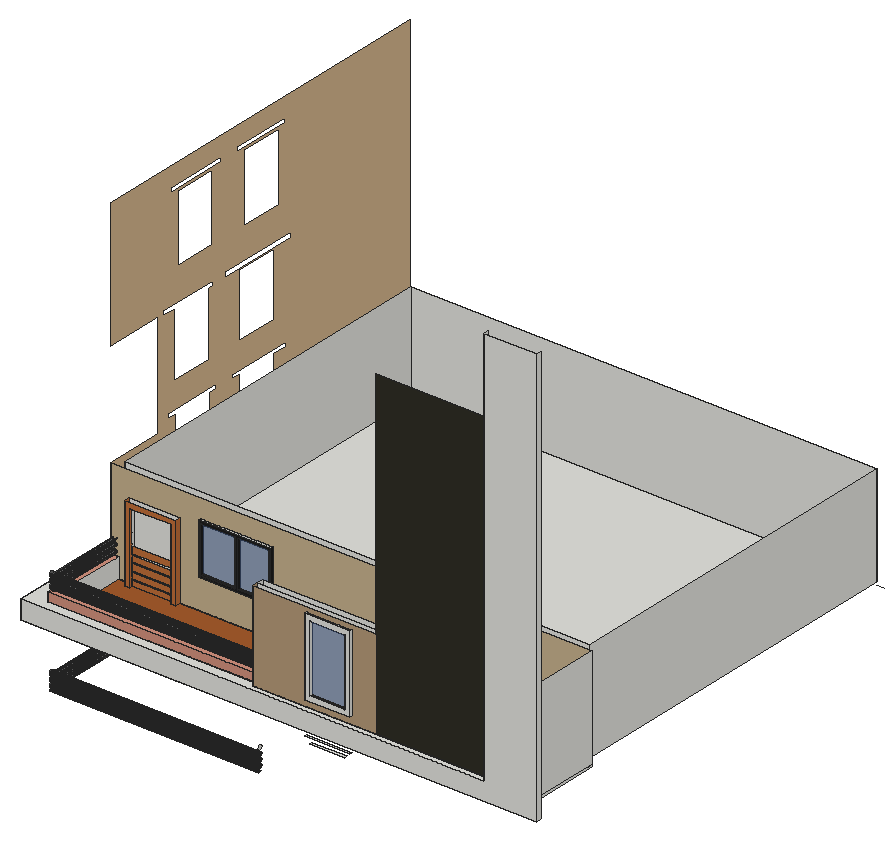
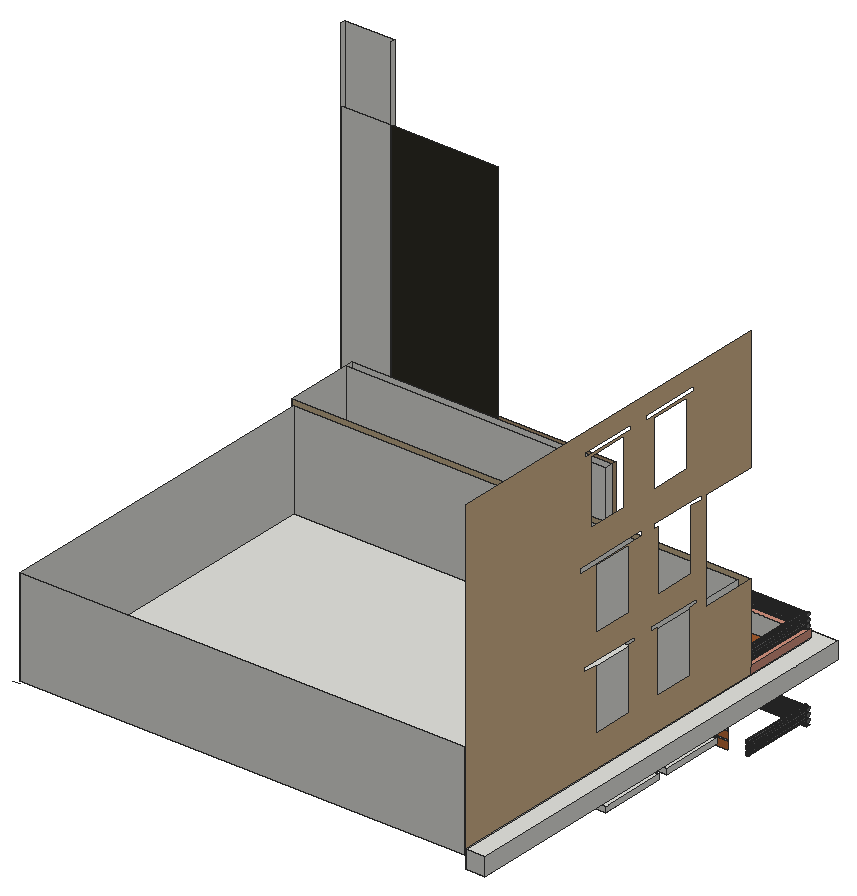
# SketchUp Ruby script. Lengths in inches.
U = 1.inch
M = Sketchup.active_model
def pt(a) = Geom::Point3d.new(a.map { |v| v * U })
def face(e, loops, mat)
  f = e.add_face(loops[0].map { |a| pt(a) })
  loops[1..].each { |l| e.add_face(l.map { |a| pt(a) }).erase! }
  f.material = f.back_material = mat if mat
  f
end
# faces: each face lists its corners as indices into pts; further lists are holes
def faces(e, pts, list, mat = nil) = list.each { |f| face(e, (f[0].is_a?(Array) ? f : [f]).map { |l| l.map { |i| pts[i] } }, mat) }
# xy, xz, yz: faces in a plane at the given z, y or x. An outline is a flat list of corners, or four numbers for a rectangle; further outlines are holes
def ring(l) = l.size == 4 ? [[l[0], l[1]], [l[2], l[1]], [l[2], l[3]], [l[0], l[3]]] : l.each_slice(2).to_a
def flat(e, list, mat, &to3) = list.each { |f| face(e, (f[0].is_a?(Array) ? f : [f]).map { |l| ring(l).map { |u, v| to3.(u, v) } }, mat) }
def xy(e, z, list, mat = nil) = flat(e, list, mat) { |x, y| [x, y, z] }
def xz(e, y, list, mat = nil) = flat(e, list, mat) { |x, z| [x, y, z] }
def yz(e, x, list, mat = nil) = flat(e, list, mat) { |y, z| [x, y, z] }
def lines(e, pts, list) = list.each { |a, b| e.add_line(pt(pts[a]), pt(pts[b])) }
# prism: a flat outline (further loops are holes) pulled along v
def prism(e, loops, v, mat = nil)
  f = face(e, loops, mat); d = Geom::Vector3d.new(v.map { |x| x * U })
  f.pushpull(f.normal.samedirection?(d) ? d.length : -d.length)
end
def box(e, o, s, mat = nil) = prism(e, [[o, [o[0] + s[0], o[1], o[2]], [o[0] + s[0], o[1] + s[1], o[2]], [o[0], o[1] + s[1], o[2]]]], [0, 0, s[2]], mat)
def at(x, y, z, deg = 0) = Geom::Transformation.translation(pt([x, y, z])) * Geom::Transformation.rotation(ORIGIN, Z_AXIS, deg.degrees)
def axes(o, x, y, z) = Geom::Transformation.new([*x, 0, *y, 0, *z, 0, *pt(o).to_a, 1])
def part(name) = M.definitions.add(name)
# library, detail: a bought-in or finely detailed component or shape, given as its bounding box
def library(name, o, s) = part(name).tap { |d| box(d.entities, o, s) }
def detail(e, o, s) = box(e.add_group.entities, o, s)
def put(e, d, t, mat = nil) = e.add_instance(d, t).tap { |i| i.material = mat if mat }
def group(e, t, mat = nil) = e.add_group.tap { |g| g.transformation = t; g.material = mat if mat }.entities
root = M.entities
M.materials.add("[0032_Moccasin]").color = [198, 177, 141]
M.materials.add("[0035_Tan]").color = [181, 154, 120]
M.materials.add("[0035_Tan]1").color = [210, 180, 140]
M.materials.add("[0134_DimGray]").color = [105, 105, 105]
M.materials.add("[Color B02]").color = [209, 145, 125]
M.materials.add("[Color M08]").color = [30, 30, 30]
M.materials.add("[Stone Coursed Rough]").color = [48, 46, 38]
M.materials.add("[Translucent Glass Blue]").color = [61, 91, 145]
M.materials["[Translucent Glass Blue]"].alpha = 0.5
M.materials.add("[Wood Square Tile 01]").color = [164, 91, 44]
M.materials.add("[Wood Veneer 01]").color = [191, 111, 58]
xy(root,456,[[66.43,116.9375,114.43,119.9375]])
xy(root,456,[[66.43,113.9375,114.43,116.9375]],"[Wood Veneer 01]")
xy(root,462,[[60.43,113.9375,120.43,119.9375]],"[Wood Veneer 01]")
xy(root,463.8125,[[144.33,116.9375,184.18,119.9375],[187.18,116.9375,224.02,119.9375]],"[Color M08]")
xy(root,464.8,[[31.875,212.29,34.875,264.41],[31.875,307.48,34.875,359.6]],"[Color M08]")
xy(root,466.8125,[[141.33,116.9375,227.02,119.9375]],"[Color M08]")
xy(root,470.15,[[352.1,17.9375,393.78,20.9375]])
xy(root,470.8,[[13.875,198.91,13.875,276.26,34.875,276.26,34.875,270.41,31.875,270.41,31.875,206.29,34.875,206.29,34.875,198.91],[13.875,289.66,13.875,372.1,34.875,372.1,34.875,365.6,31.875,365.6,31.875,301.48,34.875,301.48,34.875,289.66]])
xy(root,476.15,[[346.1,17.9375,399.78,20.9375]])
xy(root,477.3,[[13.875,198.91,34.875,276.26],[13.875,289.66,34.875,372.1]])
xy(root,483.875,[[11.5625,14.9375,11.5625,561.98,34.875,561.98,34.875,26.9375,282.125,26.9375,282.125,20.9375,623,20.9375,623,14.9375]])
xy(root,485.875,[[282.125,26.9375,604.125,35.9375]])
xy(root,489,[[34.875,26.9375,604.125,119.9375]])
xy(root,492,[[56.21,113.9375,62.21,119.9375],[110.21,113.9375,116.21,119.9375],[62.21,116.9375,110.21,119.9375],[43.875,128.9375,595.125,552.98]])
xy(root,492,[[43.875,35.9375,604.125,35.9375,604.125,119.9375,116.21,119.9375,116.21,113.9375,110.21,113.9375,110.21,116.9375,62.21,116.9375,62.21,113.9375,56.21,113.9375,56.21,119.9375,43.875,119.9375]],"[Wood Square Tile 01]")
xy(root,505.8125,[[11.5625,14.9375,561.08,14.9375,561.08,20.9375,282.125,20.9375,282.125,26.9375,34.875,26.9375,34.875,561.98,11.5625,561.98]])
xy(root,514.96,[[346.1,17.9375,399.78,20.9375]])
xy(root,516,[[282.125,26.9375,604.125,35.9375]])
xy(root,516,[[34.875,26.9375,282.125,26.9375,282.125,35.9375,43.875,35.9375,43.875,119.9375,34.875,119.9375]],"[Color B02]")
xy(root,520.96,[[352.1,17.9375,393.78,20.9375]])
xy(root,529.3125,[[141.33,116.9375,227.02,119.9375]])
xy(root,532.3125,[[144.33,116.9375,184.18,119.9375],[187.18,116.9375,224.02,119.9375]],"[Color M08]")
xz(root,14.9375,[[11.5625,483.875,623,483.875,623,980,561.08,980,561.08,505.8125,11.5625,505.8125]])
xz(root,17.9375,[[[346.1,514.96,399.78,606.77],[352.1,520.96,393.78,600.77]]])
xz(root,20.9375,[[282.125,483.875,623,492],[282.125,492,623,492,623,888,561.08,888,561.08,505.8125,282.125,505.8125],[[346.1,514.96,399.78,606.77],[352.1,520.96,393.78,600.77]]])
xz(root,20.9375,[[[282.125,505.8125,427.625,612],[346.1,514.96,399.78,606.77]]],"[0035_Tan]")
xz(root,20.9375,[[427.625,505.8125,561.08,888]],"[Stone Coursed Rough]")
xz(root,20.9375,[[352.1,520.96,393.78,600.77]],"[Translucent Glass Blue]")
xz(root,26.9375,[[34.875,483.875,282.125,489],[282.125,485.875,604.125,489],[34.875,489,282.125,505.8125],[282.125,489,604.125,492],[282.125,492,604.125,516],
  [282.125,516,604.125,612]])
xz(root,26.9375,[[34.875,505.8125,282.125,516]],"[Color B02]")
xz(root,29.17,[[37.22,519.63,41.83,519.63,41.9,520.15,41.82,520.76,41.78,520.86,37.27,520.86,37.23,520.76,37.15,520.15],[37.27,520.86,41.78,520.86,41.58,521.34,41.21,521.83,40.71,522.2,40.14,522.44,39.53,522.52,38.91,522.44,38.34,522.2,37.85,521.83,37.47,521.34]])
xz(root,29.17,[[39.53,517.77,40.14,517.85,40.71,518.09,41.21,518.47,41.58,518.96,41.82,519.53,41.83,519.63,37.22,519.63,37.23,519.53,37.47,518.96,37.85,518.47,38.34,518.09,38.91,517.85]],"[0134_DimGray]")
xz(root,35.9375,[[43.875,492,282.125,516],[282.125,492,604.125,516],[282.125,516,604.125,612]])
xz(root,113.9375,[[56.21,492,62.21,492,62.21,576,110.21,576,110.21,492,116.21,492,116.21,582,56.21,582]],"[Wood Veneer 01]")
xz(root,116.9375,[[66.43,419.66,114.43,421.37],[66.43,431.09,114.43,432.81],[66.43,442.53,114.43,444.25],[62.21,498.38,110.21,499.69],[62.21,507.45,110.21,508.75],
  [62.21,516.51,110.21,517.82],[62.21,525.57,110.21,526.88]])
xz(root,116.9375,[[[141.33,529.3125,227.02,590],[144.33,532.3125,184.18,587],[187.18,532.3125,224.02,587]]],"[Color M08]")
xz(root,116.9375,[[66.43,409.93,114.43,419.66],[66.43,421.37,114.43,431.09],[66.43,432.81,114.43,442.53],[66.43,444.25,114.43,456],[62.21,492,110.21,498.38],
  [62.21,499.69,110.21,507.45],[62.21,508.75,110.21,516.51],[62.21,517.82,110.21,525.57],[62.21,526.88,110.21,534.63]],"[Wood Veneer 01]")
xz(root,119.9375,[[56.21,486,116.21,489],[34.875,489,35.6,492],[35.6,489,56.21,492],[56.21,489,116.21,492],[116.21,489,604.125,492],
  [34.875,492,35.6,516],[35.6,492,43.875,516],[56.21,492,56.21,582,116.21,582,116.21,492,110.21,492,110.21,576,62.21,576,62.21,492],[62.21,492,110.21,576],[[141.33,529.3125,227.02,590],[144.33,532.3125,184.18,587],[187.18,532.3125,224.02,587]]])
xz(root,119.9375,[[[43.875,492,56.21,492,56.21,582,116.21,582,116.21,492,604.125,492,604.125,612,34.875,612,34.875,516,43.875,516],[141.33,529.3125,227.02,590],[39.53,517.77,38.91,517.85,38.34,518.09,37.85,518.47,37.47,518.96,37.23,519.53,37.15,520.15,37.23,520.76,37.47,521.34,37.85,521.83,38.34,522.2,38.91,522.44,39.53,522.52,40.14,522.44,40.71,522.2,41.21,521.83,41.58,521.34,41.82,520.76,41.9,520.15,41.82,519.53,41.58,518.96,41.21,518.47,40.71,518.09,40.14,517.85]]],"[0032_Moccasin]")
xz(root,119.9375,[[144.33,532.3125,184.18,587],[187.18,532.3125,224.02,587]],"[Translucent Glass Blue]")
xz(root,128.9375,[[43.875,492,595.125,612]])
xz(root,198.91,[[13.875,470.8,34.875,477.3]])
xz(root,276.26,[[13.875,470.8,34.875,477.3]])
xz(root,289.66,[[13.875,470.8,34.875,477.3]])
xz(root,372.1,[[13.875,470.8,34.875,477.3]])
xz(root,552.98,[[43.875,492,595.125,612]])
xz(root,561.98,[[11.5625,483.875,34.875,505.8125]])
yz(root,11.5625,[[14.9375,483.875,561.98,505.8125]])
yz(root,13.875,[[198.91,470.8,276.26,477.3],[289.66,470.8,372.1,477.3]])
yz(root,34.875,[[26.9375,483.875,119.9375,489],[119.9375,483.875,561.98,489],[26.9375,489,119.9375,505.8125],[119.9375,489,561.98,505.8125]])
yz(root,34.875,[[[119.9375,505.8125,119.9375,612,189.6875,612,189.6875,735.99,119.9375,735.99,119.9375,888,561.98,888,561.98,505.8125],[213.17,658.14,264.48,658.14,264.48,733.75,270.28,733.75,270.28,739.24,197.03,739.24,197.03,733.75,213.17,733.75],[309.92,546.33,361.23,546.33,361.23,621.9375,378.8,621.9375,378.8,626.625,299.55,626.625,299.55,621.9375,309.92,621.9375],[214.36,546.33,265.67,546.33,265.67,621.9375,275.92,621.9375,275.92,626.9375,204.23,626.9375,204.23,621.9375,214.36,621.9375],[219.0625,777.36,270.0625,857.18],[317.1875,777.36,368.1875,857.18],[309.92,658.14,361.23,733.75],[288.9,733.87,385.9,740.24],[208.16,859.6875,283.03,865.0625],[306.78,859.6875,378.1,865.0625]]],"[0035_Tan]1")
yz(root,34.875,[[31.46,413.06,30.85,413.14,30.27,413.375,29.78,413.75,29.4,414.24,29.17,414.82,29.09,415.43,29.17,416.04,29.4,416.62,29.78,417.11,30.27,417.49,30.85,417.72,31.46,417.81,32.08,417.72,32.65,417.49,33.14,417.11,33.52,416.62,33.76,416.04,33.84,415.43,33.76,414.82,33.52,414.24,33.14,413.75,32.65,413.375,32.08,413.14],[31.46,419.74,30.85,419.82,30.27,420.0625,29.78,420.4375,29.4,420.93,29.17,421.5,29.09,422.12,29.17,422.73,29.4,423.31,29.78,423.8,30.27,424.17,30.85,424.41,31.46,424.49,32.08,424.41,32.65,424.17,33.14,423.8,33.52,423.31,33.76,422.73,33.84,422.12,33.76,421.5,33.52,420.93,33.14,420.4375,32.65,420.0625,32.08,419.82],[31.46,426.43,30.85,426.51,30.27,426.75,29.78,427.125,29.4,427.62,29.17,428.19,29.09,428.81,29.17,429.42,29.4,429.99,29.78,430.48,30.27,430.86,30.85,431.1,31.46,431.18,32.08,431.1,32.65,430.86,33.14,430.48,33.52,429.99,33.76,429.42,33.84,428.81,33.76,428.19,33.52,427.62,33.14,427.125,32.65,426.75,32.08,426.51],[31.46,517.87,30.85,517.95,30.27,518.1875,29.78,518.5625,29.4,519.06,29.17,519.63,29.09,520.24,29.17,520.86,29.4,521.43,29.78,521.92,30.27,522.3,30.85,522.54,31.46,522.62,32.08,522.54,32.65,522.3,33.14,521.92,33.52,521.43,33.76,520.86,33.84,520.24,33.76,519.63,33.52,519.06,33.14,518.5625,32.65,518.1875,32.08,517.95],[31.46,524.62,30.85,524.7,30.27,524.9375,29.78,525.3125,29.4,525.81,29.17,526.38,29.09,526.99,29.17,527.61,29.4,528.18,29.78,528.67,30.27,529.05,30.85,529.29,31.46,529.37,32.08,529.29,32.65,529.05,33.14,528.67,33.52,528.18,33.76,527.61,33.84,526.99,33.76,526.38,33.52,525.81,33.14,525.3125,32.65,524.9375,32.08,524.7],
  [31.46,531.37,30.85,531.45,30.27,531.6875,29.78,532.0625,29.4,532.56,29.17,533.13,29.09,533.74,29.17,534.36,29.4,534.93,29.78,535.42,30.27,535.8,30.85,536.04,31.46,536.12,32.08,536.04,32.65,535.8,33.14,535.42,33.52,534.93,33.76,534.36,33.84,533.74,33.76,533.13,33.52,532.56,33.14,532.0625,32.65,531.6875,32.08,531.45]],"[0134_DimGray]")
yz(root,34.875,[[26.9375,505.8125,119.9375,516]],"[Color B02]")
yz(root,43.875,[[35.9375,492,119.9375,516],[128.9375,492,552.98,612]])
yz(root,56.21,[[113.9375,492,119.9375,582]],"[Wood Veneer 01]")
yz(root,62.21,[[116.9375,492,119.9375,576]])
yz(root,62.21,[[113.9375,492,116.9375,576]],"[Wood Veneer 01]")
yz(root,110.21,[[116.9375,492,119.9375,576]])
yz(root,110.21,[[113.9375,492,116.9375,576]],"[Wood Veneer 01]")
yz(root,116.21,[[113.9375,492,119.9375,582]],"[Wood Veneer 01]")
yz(root,141.33,[[116.9375,529.3125,119.9375,590]],"[Color M08]")
yz(root,144.33,[[116.9375,532.3125,119.9375,587]],"[Color M08]")
yz(root,184.18,[[116.9375,532.3125,119.9375,587]],"[Color M08]")
yz(root,187.18,[[116.9375,532.3125,119.9375,587]],"[Color M08]")
yz(root,224.02,[[116.9375,532.3125,119.9375,587]],"[Color M08]")
yz(root,227.02,[[116.9375,529.3125,119.9375,590]],"[Color M08]")
yz(root,282.125,[[31.46,433.12,30.85,433.2,30.27,433.4375,29.78,433.8125,29.4,434.31,29.17,434.88,29.09,435.49,29.17,436.11,29.4,436.68,29.78,437.17,30.27,437.55,30.85,437.79,31.46,437.87,32.08,437.79,32.65,437.55,33.14,437.17,33.52,436.68,33.76,436.11,33.84,435.49,33.76,434.88,33.52,434.31,33.14,433.8125,32.65,433.4375,32.08,433.2],[20.9375,483.875,26.9375,492],[26.9375,483.875,35.9375,485.875],[20.9375,492,26.9375,505.8125],[[26.9375,516,35.9375,612],[31.46,524.62,32.08,524.7,32.65,524.9375,33.14,525.3125,33.52,525.81,33.76,526.38,33.84,526.99,33.76,527.61,33.52,528.18,33.14,528.67,32.65,529.05,32.08,529.29,31.46,529.37,30.85,529.29,30.27,529.05,29.78,528.67,29.4,528.18,29.17,527.61,29.09,526.99,29.17,526.38,29.4,525.81,29.78,525.3125,30.27,524.9375,30.85,524.7],[31.46,531.37,32.08,531.45,32.65,531.6875,33.14,532.0625,33.52,532.56,33.76,533.13,33.84,533.74,33.76,534.36,33.52,534.93,33.14,535.42,32.65,535.8,32.08,536.04,31.46,536.12,30.85,536.04,30.27,535.8,29.78,535.42,29.4,534.93,29.17,534.36,29.09,533.74,29.17,533.13,29.4,532.56,29.78,532.0625,30.27,531.6875,30.85,531.45],[31.46,538.12,32.08,538.2,32.65,538.4375,33.14,538.8125,33.52,539.31,33.76,539.88,33.84,540.49,33.76,541.11,33.52,541.68,33.14,542.17,32.65,542.55,32.08,542.79,31.46,542.87,30.85,542.79,30.27,542.55,29.78,542.17,29.4,541.68,29.17,541.11,29.09,540.49,29.17,539.88,29.4,539.31,29.78,538.8125,30.27,538.4375,30.85,538.2],[31.46,544.87,32.08,544.95,32.65,545.1875,33.14,545.5625,33.52,546.06,33.76,546.63,33.84,547.24,33.76,547.86,33.52,548.43,33.14,548.92,32.65,549.3,32.08,549.54,31.46,549.62,30.85,549.54,30.27,549.3,29.78,548.92,29.4,548.43,29.17,547.86,29.09,547.24,29.17,546.63,29.4,546.06,29.78,545.5625,30.27,545.1875,30.85,544.95],[31.46,517.87,32.08,517.95,32.65,518.1875,33.14,518.5625,33.52,519.06,33.76,519.63,33.84,520.24,33.76,520.86,33.52,521.43,33.14,521.92,32.65,522.3,32.08,522.54,31.46,522.62,30.85,522.54,30.27,522.3,29.78,521.92,29.4,521.43,29.17,520.86,29.09,520.24,29.17,519.63,29.4,519.06,29.78,518.5625,30.27,518.1875,30.85,517.95]]])
yz(root,282.125,[[20.9375,505.8125,26.9375,612]],"[0035_Tan]")
yz(root,346.1,[[17.9375,514.96,20.9375,606.77]])
yz(root,352.1,[[17.9375,520.96,20.9375,600.77]])
yz(root,393.78,[[17.9375,520.96,20.9375,600.77]])
yz(root,399.78,[[17.9375,514.96,20.9375,606.77]])
yz(root,561.08,[[14.9375,505.8125,20.9375,980]])
yz(root,595.125,[[128.9375,492,552.98,612]])
yz(root,604.125,[[26.9375,489,119.9375,492],[26.9375,492,35.9375,516],[35.9375,492,119.9375,612],[26.9375,516,35.9375,612]])
yz(root,623,[[14.9375,483.875,20.9375,980]])
p = [[282.125,29.4,409.93],[282.125,29.78,410.42],[34.875,29.78,410.42],[34.875,29.4,409.93],[282.125,33.14,410.42],[282.125,33.52,409.93],
  [34.875,33.52,409.93],[34.875,33.14,410.42],[282.125,30.27,410.8],[34.875,30.27,410.8],[282.125,32.65,410.8],[34.875,32.65,410.8],
  [282.125,30.85,411.04],[34.875,30.85,411.04],[282.125,32.08,411.04],[34.875,32.08,411.04],[282.125,31.46,411.12],[34.875,31.46,411.12],
  [282.125,30.85,413.14],[282.125,30.27,413.375],[34.875,30.27,413.375],[34.875,30.85,413.14],[282.125,31.46,413.06],[34.875,31.46,413.06],
  [282.125,32.08,413.14],[34.875,32.08,413.14],[282.125,32.65,413.375],[34.875,32.65,413.375],[282.125,29.78,413.75],[34.875,29.78,413.75],
  [282.125,33.14,413.75],[34.875,33.14,413.75],[38.89,119.9375,413.82],[39.51,119.9375,413.74],[39.51,29.25,413.74],[38.89,29.25,413.82],
  [40.12,119.9375,413.82],[40.12,29.25,413.82],[38.32,119.9375,414.06],[38.32,29.25,414.06],[40.69,119.9375,414.06],[40.69,29.25,414.06],
  [282.125,29.4,414.24],[34.875,29.4,414.24],[282.125,33.52,414.24],[34.875,33.52,414.24],[37.83,119.9375,414.43],[37.83,29.25,414.43],
  [41.1875,119.9375,414.43],[41.1875,29.25,414.43],[282.125,29.17,414.82],[34.875,29.17,414.82],[282.125,33.76,414.82],[34.875,33.76,414.82],
  [37.45,119.9375,414.92],[37.45,29.25,414.92],[41.5625,119.9375,414.92],[41.5625,29.25,414.92],[282.125,29.09,415.43],[34.875,29.09,415.43],
  [282.125,33.84,415.43],[34.875,33.84,415.43],[37.21,119.9375,415.5],[37.21,29.25,415.5],[41.8,119.9375,415.5],[41.8,29.25,415.5],
  [282.125,29.17,416.04],[34.875,29.17,416.04],[282.125,33.76,416.04],[34.875,33.76,416.04],[37.13,119.9375,416.11],[37.13,29.25,416.11],
  [41.88,119.9375,416.11],[41.88,29.25,416.11],[282.125,29.4,416.62],[34.875,29.4,416.62],[282.125,33.52,416.62],[34.875,33.52,416.62],
  [37.21,119.9375,416.73],[37.21,29.25,416.73],[41.8,119.9375,416.73],[41.8,29.25,416.73],[282.125,29.78,417.11],[34.875,29.78,417.11],
  [282.125,33.14,417.11],[34.875,33.14,417.11],[37.45,119.9375,417.3],[37.45,29.25,417.3],[41.5625,119.9375,417.3],[41.5625,29.25,417.3],
  [282.125,30.27,417.49],[34.875,30.27,417.49],[282.125,32.65,417.49],[34.875,32.65,417.49],[37.83,119.9375,417.79],[37.83,29.25,417.79],
  [41.1875,119.9375,417.79],[41.1875,29.25,417.79],[282.125,30.85,417.72],[34.875,30.85,417.72],[282.125,32.08,417.72],[34.875,32.08,417.72],
  [282.125,31.46,417.81],[34.875,31.46,417.81],[38.32,119.9375,418.17],[38.32,29.25,418.17],[40.69,119.9375,418.17],[40.69,29.25,418.17],
  [38.89,119.9375,418.41],[38.89,29.25,418.41],[40.12,119.9375,418.41],[40.12,29.25,418.41],[39.51,119.9375,418.49],[39.51,29.25,418.49],
  [282.125,31.46,419.74],[282.125,30.85,419.82],[34.875,30.85,419.82],[34.875,31.46,419.74],[282.125,32.08,419.82],[34.875,32.08,419.82],
  [282.125,30.27,420.0625],[34.875,30.27,420.0625],[282.125,32.65,420.0625],[34.875,32.65,420.0625],[282.125,29.78,420.4375],[34.875,29.78,420.4375],
  [282.125,33.14,420.4375],[34.875,33.14,420.4375],[38.89,119.9375,420.26],[39.51,119.9375,420.17],[39.51,29.25,420.17],[38.89,29.25,420.26],
  [40.12,119.9375,420.26],[40.12,29.25,420.26],[38.32,119.9375,420.49],[38.32,29.25,420.49],[40.69,119.9375,420.49],[40.69,29.25,420.49],
  [282.125,29.4,420.93],[34.875,29.4,420.93],[282.125,33.52,420.93],[34.875,33.52,420.93],[37.83,119.9375,420.87],[37.83,29.25,420.87],
  [41.1875,119.9375,420.87],[41.1875,29.25,420.87],[282.125,29.17,421.5],[34.875,29.17,421.5],[37.45,119.9375,421.36],[37.45,29.25,421.36],
  [41.5625,119.9375,421.36],[41.5625,29.25,421.36],[282.125,33.76,421.5],[34.875,33.76,421.5],[37.21,119.9375,421.93],[37.21,29.25,421.93],
  [41.8,119.9375,421.93],[41.8,29.25,421.93],[282.125,29.09,422.12],[34.875,29.09,422.12],[282.125,33.84,422.12],[34.875,33.84,422.12],
  [37.13,119.9375,422.55],[37.13,29.25,422.55],[41.88,119.9375,422.55],[41.88,29.25,422.55],[282.125,29.17,422.73],[34.875,29.17,422.73],
  [282.125,33.76,422.73],[34.875,33.76,422.73],[37.21,119.9375,423.16],[37.21,29.25,423.16],[41.8,119.9375,423.16],[41.8,29.25,423.16],
  [282.125,29.4,423.31],[34.875,29.4,423.31],[282.125,33.52,423.31],[34.875,33.52,423.31],[37.45,119.9375,423.74],[37.45,29.25,423.74],
  [41.5625,119.9375,423.74],[41.5625,29.25,423.74],[282.125,29.78,423.8],[34.875,29.78,423.8],[282.125,33.14,423.8],[34.875,33.14,423.8],
  [37.83,119.9375,424.23],[37.83,29.25,424.23],[41.1875,119.9375,424.23],[41.1875,29.25,424.23],[282.125,30.27,424.17],[34.875,30.27,424.17],
  [282.125,32.65,424.17],[34.875,32.65,424.17],[38.32,119.9375,424.61],[38.32,29.25,424.61],[40.69,119.9375,424.61],[40.69,29.25,424.61],
  [282.125,30.85,424.41],[34.875,30.85,424.41],[282.125,32.08,424.41],[34.875,32.08,424.41],[282.125,31.46,424.49],[34.875,31.46,424.49],
  [38.89,119.9375,424.84],[38.89,29.25,424.84],[40.12,119.9375,424.84],[40.12,29.25,424.84],[39.51,119.9375,424.92],[39.51,29.25,424.92],
  [282.125,31.46,426.43],[282.125,30.85,426.51],[34.875,30.85,426.51],[34.875,31.46,426.43],[282.125,32.08,426.51],[34.875,32.08,426.51],
  [38.89,119.9375,426.57],[39.51,119.9375,426.49],[39.51,29.25,426.49],[38.89,29.25,426.57],[40.12,119.9375,426.57],[40.12,29.25,426.57],
  [282.125,30.27,426.75],[34.875,30.27,426.75],[282.125,32.65,426.75],[34.875,32.65,426.75],[38.32,119.9375,426.81],[38.32,29.25,426.81],
  [40.69,119.9375,426.81],[40.69,29.25,426.81],[282.125,29.78,427.125],[34.875,29.78,427.125],[282.125,33.14,427.125],[34.875,33.14,427.125],
  [37.83,119.9375,427.18],[37.83,29.25,427.18],[41.1875,119.9375,427.18],[41.1875,29.25,427.18],[282.125,29.4,427.62],[34.875,29.4,427.62],
  [282.125,33.52,427.62],[34.875,33.52,427.62],[37.45,119.9375,427.67],[37.45,29.25,427.67],[41.5625,119.9375,427.67],[41.5625,29.25,427.67],
  [282.125,29.17,428.19],[34.875,29.17,428.19],[282.125,33.76,428.19],[34.875,33.76,428.19],[37.21,119.9375,428.25],[37.21,29.25,428.25],
  [41.8,119.9375,428.25],[41.8,29.25,428.25],[282.125,29.09,428.81],[34.875,29.09,428.81],[37.13,119.9375,428.86],[37.13,29.25,428.86],
  [41.88,119.9375,428.86],[41.88,29.25,428.86],[282.125,33.84,428.81],[34.875,33.84,428.81],[282.125,29.17,429.42],[34.875,29.17,429.42],
  [282.125,33.76,429.42],[34.875,33.76,429.42],[37.21,119.9375,429.48],[37.21,29.25,429.48],[41.8,119.9375,429.48],[41.8,29.25,429.48],
  [282.125,29.4,429.99],[34.875,29.4,429.99],[282.125,33.52,429.99],[34.875,33.52,429.99],[37.45,119.9375,430.05],[37.45,29.25,430.05],
  [41.5625,119.9375,430.05],[41.5625,29.25,430.05],[37.83,119.9375,430.54],[37.83,29.25,430.54],[41.1875,119.9375,430.54],[41.1875,29.25,430.54],
  [282.125,29.78,430.48],[34.875,29.78,430.48],[282.125,33.14,430.48],[34.875,33.14,430.48],[38.32,119.9375,430.92],[38.32,29.25,430.92],
  [40.69,119.9375,430.92],[40.69,29.25,430.92],[282.125,30.27,430.86],[34.875,30.27,430.86],[282.125,32.65,430.86],[34.875,32.65,430.86],
  [38.89,119.9375,431.16],[38.89,29.25,431.16],[40.12,119.9375,431.16],[40.12,29.25,431.16],[282.125,30.85,431.1],[34.875,30.85,431.1],
  [282.125,32.08,431.1],[34.875,32.08,431.1],[282.125,31.46,431.18],[34.875,31.46,431.18],[39.51,119.9375,431.24],[39.51,29.25,431.24],
  [38.91,119.9375,517.85],[39.53,119.9375,517.77],[39.53,29.17,517.77],[38.91,29.17,517.85],[40.14,119.9375,517.85],[40.14,29.17,517.85],
  [38.34,119.9375,518.09],[38.34,29.17,518.09],[40.71,119.9375,518.09],[40.71,29.17,518.09],[282.125,30.85,517.95],[282.125,30.27,518.1875],
  [34.875,30.27,518.1875],[34.875,30.85,517.95],[282.125,31.46,517.87],[34.875,31.46,517.87],[282.125,32.08,517.95],[34.875,32.08,517.95],
  [282.125,32.65,518.1875],[34.875,32.65,518.1875],[37.85,119.9375,518.47],[37.85,29.17,518.47],[41.21,119.9375,518.47],[41.21,29.17,518.47],
  [282.125,29.78,518.5625],[34.875,29.78,518.5625],[282.125,33.14,518.5625],[34.875,33.14,518.5625],[37.47,119.9375,518.96],[37.47,29.17,518.96],
  [41.58,119.9375,518.96],[41.58,29.17,518.96],[282.125,29.4,519.06],[34.875,29.4,519.06],[282.125,33.52,519.06],[34.875,33.52,519.06],
  [37.23,119.9375,519.53],[37.23,29.17,519.53],[41.82,119.9375,519.53],[41.82,29.17,519.53],[282.125,29.17,519.63],[41.83,29.17,519.63],
  [37.22,29.17,519.63],[34.875,29.17,519.63],[282.125,33.76,519.63],[34.875,33.76,519.63],[37.15,119.9375,520.15],[37.15,29.17,520.15],
  [41.9,119.9375,520.15],[41.9,29.17,520.15],[282.125,29.09,520.24],[34.875,29.09,520.24],[282.125,33.84,520.24],[34.875,33.84,520.24],
  [37.23,119.9375,520.76],[37.23,29.17,520.76],[41.82,119.9375,520.76],[41.82,29.17,520.76],[282.125,29.17,520.86],[41.78,29.17,520.86],
  [37.27,29.17,520.86],[34.875,29.17,520.86],[282.125,33.76,520.86],[34.875,33.76,520.86],[37.47,119.9375,521.34],[37.47,29.17,521.34],
  [41.58,119.9375,521.34],[41.58,29.17,521.34],[282.125,29.4,521.43],[34.875,29.4,521.43],[282.125,33.52,521.43],[34.875,33.52,521.43],
  [37.85,119.9375,521.83],[37.85,29.17,521.83],[41.21,119.9375,521.83],[41.21,29.17,521.83],[282.125,29.78,521.92],[34.875,29.78,521.92],
  [282.125,33.14,521.92],[34.875,33.14,521.92],[38.34,119.9375,522.2],[38.34,29.17,522.2],[40.71,119.9375,522.2],[40.71,29.17,522.2],
  [282.125,30.27,522.3],[34.875,30.27,522.3],[282.125,32.65,522.3],[34.875,32.65,522.3],[38.91,119.9375,522.44],[38.91,29.17,522.44],
  [40.14,119.9375,522.44],[40.14,29.17,522.44],[282.125,30.85,522.54],[34.875,30.85,522.54],[282.125,32.08,522.54],[34.875,32.08,522.54],
  [39.53,119.9375,522.52],[39.53,29.17,522.52],[282.125,31.46,522.62],[34.875,31.46,522.62],[282.125,31.46,524.62],[282.125,30.85,524.7],
  [34.875,30.85,524.7],[34.875,31.46,524.62],[282.125,32.08,524.7],[34.875,32.08,524.7],[282.125,30.27,524.9375],[34.875,30.27,524.9375],
  [282.125,32.65,524.9375],[34.875,32.65,524.9375],[282.125,29.78,525.3125],[34.875,29.78,525.3125],[282.125,33.14,525.3125],[34.875,33.14,525.3125],
  [38.91,119.9375,525.42],[39.53,119.9375,525.34],[39.53,29.17,525.34],[38.91,29.17,525.42],[40.14,119.9375,525.42],[40.14,29.17,525.42],
  [282.125,29.4,525.81],[34.875,29.4,525.81],[282.125,33.52,525.81],[34.875,33.52,525.81],[38.34,119.9375,525.65],[38.34,29.17,525.65],
  [40.71,119.9375,525.65],[40.71,29.17,525.65],[37.85,119.9375,526.03],[37.85,29.17,526.03],[41.21,119.9375,526.03],[41.21,29.17,526.03],
  [282.125,29.17,526.38],[41.47,29.17,526.38],[37.58,29.17,526.38],[34.875,29.17,526.38],[282.125,33.76,526.38],[34.875,33.76,526.38],
  [37.47,119.9375,526.52],[37.47,29.17,526.52],[41.58,119.9375,526.52],[41.58,29.17,526.52],[282.125,29.09,526.99],[34.875,29.09,526.99],
  [282.125,33.84,526.99],[34.875,33.84,526.99],[37.23,119.9375,527.1],[37.23,29.17,527.1],[41.82,119.9375,527.1],[41.82,29.17,527.1],
  [282.125,29.17,527.61],[41.89,29.17,527.61],[37.17,29.17,527.61],[34.875,29.17,527.61],[282.125,33.76,527.61],[34.875,33.76,527.61],
  [37.15,119.9375,527.71],[37.22,29.17,527.19],[37.15,29.17,527.71],[41.9,119.9375,527.71],[41.9,29.17,527.71],[41.83,29.17,527.19],
  [282.125,29.4,528.18],[34.875,29.4,528.18],[282.125,33.52,528.18],[34.875,33.52,528.18],[37.23,119.9375,528.32],[37.23,29.17,528.32],
  [41.82,119.9375,528.32],[41.82,29.17,528.32],[282.125,29.78,528.67],[34.875,29.78,528.67],[282.125,33.14,528.67],[34.875,33.14,528.67],
  [37.47,119.9375,528.9],[37.27,29.17,528.42],[37.47,29.17,528.9],[41.58,119.9375,528.9],[41.58,29.17,528.9],[41.78,29.17,528.42],
  [282.125,30.27,529.05],[34.875,30.27,529.05],[282.125,32.65,529.05],[34.875,32.65,529.05],[37.85,119.9375,529.39],[37.85,29.17,529.39],
  [41.21,119.9375,529.39],[41.21,29.17,529.39],[282.125,30.85,529.29],[34.875,30.85,529.29],[282.125,32.08,529.29],[34.875,32.08,529.29],
  [282.125,31.46,529.37],[34.875,31.46,529.37],[38.34,119.9375,529.77],[38.34,29.17,529.77],[40.71,119.9375,529.77],[40.71,29.17,529.77],
  [38.91,119.9375,530],[38.91,29.17,530],[40.14,119.9375,530],[40.14,29.17,530],[39.53,119.9375,530.09],[39.53,29.17,530.09],
  [282.125,30.85,531.45],[282.125,30.27,531.6875],[34.875,30.27,531.6875],[34.875,30.85,531.45],[282.125,31.46,531.37],[34.875,31.46,531.37],
  [282.125,32.08,531.45],[34.875,32.08,531.45],[282.125,32.65,531.6875],[34.875,32.65,531.6875],[282.125,29.78,532.0625],[34.875,29.78,532.0625],
  [282.125,33.14,532.0625],[34.875,33.14,532.0625],[38.91,119.9375,532.17],[39.53,119.9375,532.09],[39.53,29.17,532.09],[38.91,29.17,532.17],
  [40.14,119.9375,532.17],[40.14,29.17,532.17],[282.125,29.4,532.56],[34.875,29.4,532.56],[282.125,33.52,532.56],[34.875,33.52,532.56],
  [38.34,119.9375,532.4],[38.34,29.17,532.4],[40.71,119.9375,532.4],[40.71,29.17,532.4],[37.85,119.9375,532.78],[37.85,29.17,532.78],
  [41.21,119.9375,532.78],[41.21,29.17,532.78],[282.125,29.17,533.13],[41.47,29.17,533.13],[37.58,29.17,533.13],[34.875,29.17,533.13],
  [282.125,33.76,533.13],[34.875,33.76,533.13],[37.47,119.9375,533.27],[37.47,29.17,533.27],[41.58,119.9375,533.27],[41.58,29.17,533.27],
  [282.125,29.09,533.74],[34.875,29.09,533.74],[282.125,33.84,533.74],[34.875,33.84,533.74],[37.23,119.9375,533.85],[37.23,29.17,533.85],
  [41.82,119.9375,533.85],[41.82,29.17,533.85],[282.125,29.17,534.36],[41.89,29.17,534.36],[37.17,29.17,534.36],[34.875,29.17,534.36],
  [282.125,33.76,534.36],[34.875,33.76,534.36],[37.15,119.9375,534.46],[37.22,29.17,533.94],[37.15,29.17,534.46],[41.9,119.9375,534.46],
  [41.9,29.17,534.46],[41.83,29.17,533.94],[595.125,552.98,489],[604.125,552.98,489]]
faces(root,p,[[0,1,2,3],[4,5,6,7],[1,8,9,2],[10,4,7,11],[8,12,13,9],[14,10,11,15],[12,16,17,13],[16,14,15,17],
  [18,19,20,21],[22,18,21,23],[24,22,23,25],[26,24,25,27],[19,28,29,20],[30,26,27,31],[32,33,34,35],[33,36,37,34],
  [38,32,35,39],[36,40,41,37],[28,42,43,29],[44,30,31,45],[46,38,39,47],[40,48,49,41],[42,50,51,43],[52,44,45,53],
  [54,46,47,55],[48,56,57,49],[50,58,59,51],[60,52,53,61],[62,54,55,63],[56,64,65,57],[58,66,67,59],[68,60,61,69],
  [70,62,63,71],[64,72,73,65],[66,74,75,67],[76,68,69,77],[78,70,71,79],[72,80,81,73],[74,82,83,75],[84,76,77,85],
  [86,78,79,87],[80,88,89,81],[82,90,91,83],[92,84,85,93],[94,86,87,95],[88,96,97,89],[90,98,99,91],[100,92,93,101],
  [98,102,103,99],[102,100,101,103],[104,94,95,105],[96,106,107,97],[108,104,105,109],[106,110,111,107],[112,108,109,113],[110,112,113,111],
  [114,115,116,117],[118,114,117,119],[115,120,121,116],[122,118,119,123],[120,124,125,121],[126,122,123,127],[128,129,130,131],[129,132,133,130],
  [134,128,131,135],[132,136,137,133],[124,138,139,125],[140,126,127,141],[142,134,135,143],[136,144,145,137],[138,146,147,139],[148,142,143,149],
  [144,150,151,145],[152,140,141,153],[154,148,149,155],[150,156,157,151],[146,158,159,147],[160,152,153,161],[162,154,155,163],[156,164,165,157],
  [158,166,167,159],[168,160,161,169],[170,162,163,171],[164,172,173,165],[166,174,175,167],[176,168,169,177],[178,170,171,179],[172,180,181,173],
  [174,182,183,175],[184,176,177,185],[186,178,179,187],[180,188,189,181],[182,190,191,183],[192,184,185,193],[194,186,187,195],[188,196,197,189],
  [190,198,199,191],[200,192,193,201],[198,202,203,199],[202,200,201,203],[204,194,195,205],[196,206,207,197],[208,204,205,209],[206,208,209,207],
  [210,211,212,213],[214,210,213,215],[216,217,218,219],[217,220,221,218],[211,222,223,212],[224,214,215,225],[226,216,219,227],[220,228,229,221],
  [222,230,231,223],[232,224,225,233],[234,226,227,235],[228,236,237,229],[230,238,239,231],[240,232,233,241],[242,234,235,243],[236,244,245,237],
  [238,246,247,239],[248,240,241,249],[250,242,243,251],[244,252,253,245],[246,254,255,247],[256,250,251,257],[252,258,259,253],[260,248,249,261],
  [254,262,263,255],[264,260,261,265],[266,256,257,267],[258,268,269,259],[262,270,271,263],[272,264,265,273],[274,266,267,275],[268,276,277,269],
  [278,274,275,279],[276,280,281,277],[270,282,283,271],[284,272,273,285],[286,278,279,287],[280,288,289,281],[282,290,291,283],[292,284,285,293],
  [294,286,287,295],[288,296,297,289],[290,298,299,291],[300,292,293,301],[298,302,303,299],[302,300,301,303],[304,294,295,305],[296,304,305,297],
  [306,307,308,309],[307,310,311,308],[312,306,309,313],[310,314,315,311],[316,317,318,319],[320,316,319,321],[322,320,321,323],[324,322,323,325],
  [326,312,313,327],[314,328,329,315],[317,330,331,318],[332,324,325,333],[334,326,327,335],[328,336,337,329],[330,338,339,331],[340,332,333,341],
  [342,334,335,343],[336,344,345,337],[338,346,347,348,349,339],[350,340,341,351],[352,342,343,348,353],[344,354,355,347,345],[346,356,357,349,348,347],[358,350,351,359],
  [360,352,353,361],[354,362,363,355],[356,364,365,366,367,357],[368,358,359,369],[370,360,361,366,371],[362,372,373,365,363],[364,374,375,367,366,365],[376,368,369,377],
  [378,370,371,379],[372,380,381,373],[374,382,383,375],[384,376,377,385],[386,378,379,387],[380,388,389,381],[382,390,391,383],[392,384,385,393],
  [394,386,387,395],[388,396,397,389],[390,398,399,391],[400,392,393,401],[402,394,395,403],[396,402,403,397],[398,404,405,399],[404,400,401,405],
  [406,407,408,409],[410,406,409,411],[407,412,413,408],[414,410,411,415],[412,416,417,413],[418,414,415,419],[420,421,422,423],[421,424,425,422],
  [416,426,427,417],[428,418,419,429],[430,420,423,431],[424,432,433,425],[434,430,431,435],[432,436,437,433],[426,438,439,440,441,427],[442,428,429,443],
  [444,434,435,440,445],[436,446,447,439,437],[438,448,449,441,440,439],[450,442,443,451],[452,444,445,453],[446,454,455,447],[448,456,457,458,459,449],[460,450,451,461],
  [462,452,453,463,458,464],[454,465,466,457,467,455],[456,468,469,459,458,457],[470,460,461,471],[472,462,464,473],[465,474,475,466],[468,476,477,469],[478,470,471,479],
  [480,472,473,481,482],[474,483,484,485,475],[476,486,487,477],[488,478,479,489],[490,480,482,491],[483,492,493,484],[486,494,495,487],[496,488,489,497],
  [494,498,499,495],[498,496,497,499],[500,490,491,501],[492,502,503,493],[504,500,501,505],[502,506,507,503],[508,504,505,509],[506,508,509,507],
  [510,511,512,513],[514,510,513,515],[516,514,515,517],[518,516,517,519],[511,520,521,512],[522,518,519,523],[524,525,526,527],[525,528,529,526],
  [520,530,531,521],[532,522,523,533],[534,524,527,535],[528,536,537,529],[538,534,535,539],[536,540,541,537],[530,542,543,544,545,531],[546,532,533,547],
  [548,538,539,544,549],[540,550,551,543,541],[542,552,553,545,544,543],[554,546,547,555],[556,548,549,557],[550,558,559,551],[552,560,561,562,563,553],[564,554,555,565],
  [566,556,557,567,562,568],[558,569,570,561,571,559]],"[0134_DimGray]")
lines(root,p,[[572,573]])
